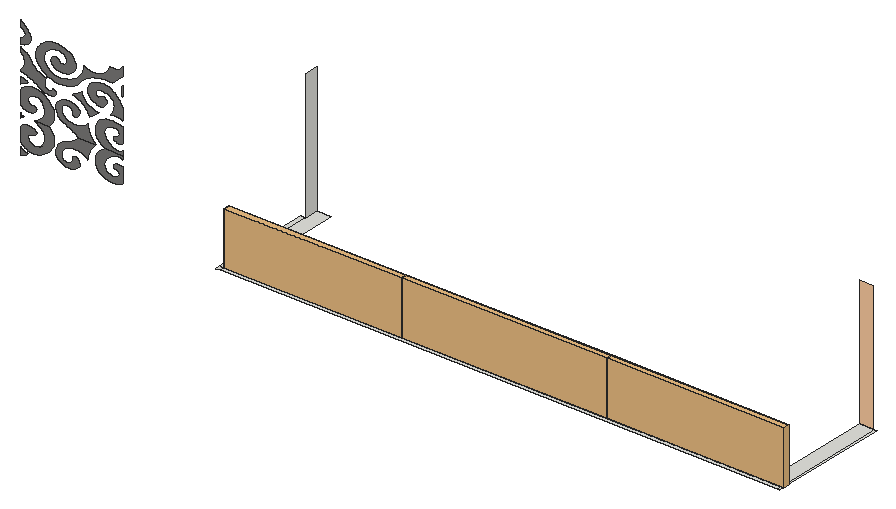
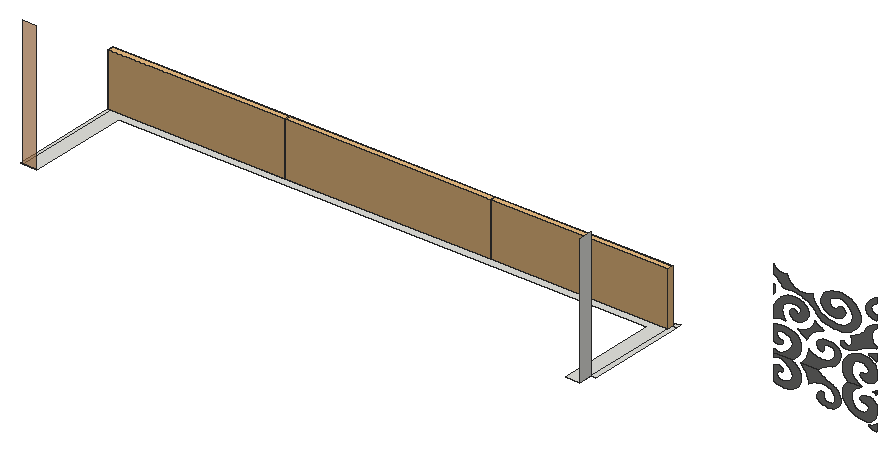
# SketchUp Ruby script. Lengths in inches.
U = 1.inch
M = Sketchup.active_model
def pt(a) = Geom::Point3d.new(a.map { |v| v * U })
def face(e, loops, mat)
  f = e.add_face(loops[0].map { |a| pt(a) })
  loops[1..].each { |l| e.add_face(l.map { |a| pt(a) }).erase! }
  f.material = f.back_material = mat if mat
  f
end
# faces: each face lists its corners as indices into pts; further lists are holes
def faces(e, pts, list, mat = nil) = list.each { |f| face(e, (f[0].is_a?(Array) ? f : [f]).map { |l| l.map { |i| pts[i] } }, mat) }
# xy, xz, yz: faces in a plane at the given z, y or x. An outline is a flat list of corners, or four numbers for a rectangle; further outlines are holes
def ring(l) = l.size == 4 ? [[l[0], l[1]], [l[2], l[1]], [l[2], l[3]], [l[0], l[3]]] : l.each_slice(2).to_a
def flat(e, list, mat, &to3) = list.each { |f| face(e, (f[0].is_a?(Array) ? f : [f]).map { |l| ring(l).map { |u, v| to3.(u, v) } }, mat) }
def xy(e, z, list, mat = nil) = flat(e, list, mat) { |x, y| [x, y, z] }
def xz(e, y, list, mat = nil) = flat(e, list, mat) { |x, z| [x, y, z] }
def yz(e, x, list, mat = nil) = flat(e, list, mat) { |y, z| [x, y, z] }
def lines(e, pts, list) = list.each { |a, b| e.add_line(pt(pts[a]), pt(pts[b])) }
# prism: a flat outline (further loops are holes) pulled along v
def prism(e, loops, v, mat = nil)
  f = face(e, loops, mat); d = Geom::Vector3d.new(v.map { |x| x * U })
  f.pushpull(f.normal.samedirection?(d) ? d.length : -d.length)
end
def box(e, o, s, mat = nil) = prism(e, [[o, [o[0] + s[0], o[1], o[2]], [o[0] + s[0], o[1] + s[1], o[2]], [o[0], o[1] + s[1], o[2]]]], [0, 0, s[2]], mat)
def at(x, y, z, deg = 0) = Geom::Transformation.translation(pt([x, y, z])) * Geom::Transformation.rotation(ORIGIN, Z_AXIS, deg.degrees)
def axes(o, x, y, z) = Geom::Transformation.new([*x, 0, *y, 0, *z, 0, *pt(o).to_a, 1])
def part(name) = M.definitions.add(name)
# library, detail: a bought-in or finely detailed component or shape, given as its bounding box
def library(name, o, s) = part(name).tap { |d| box(d.entities, o, s) }
def detail(e, o, s) = box(e.add_group.entities, o, s)
def put(e, d, t, mat = nil) = e.add_instance(d, t).tap { |i| i.material = mat if mat }
def group(e, t, mat = nil) = e.add_group.tap { |g| g.transformation = t; g.material = mat if mat }.entities
root = M.entities
M.materials.add("[0043_SaddleBrown]4").color = [124, 123, 122]
M.materials.add("[Granite Light Gray]").color = [149, 148, 144]
M.materials.add("[Wood Floor]").color = [224, 152, 88]
M.materials["[Wood Floor]"].alpha = 0.68
c1 = library("Glass Railing",[0,0,0],[139.5,4.76,42])
xy(root,293,[[548.32,556.4375,551.76,559.875],[551.76,556.4375,990.19,559.875],[990.19,556.4375,992.12,559.875],[548.32,559.875,551.76,640.11],[551.76,559.875,990.19,559.875,990.19,651.03,978.86,651.03,978.86,571.2,563.08,571.2,563.08,651.03,551.76,651.03],
  [990.19,559.875,992.12,651.03]])
xz(root,589.17,[[367.98,295.77,367.98,301,368.33,300.64,368.72,300.3,369.14,299.98,369.59,299.68,370.0625,299.4,370.5625,299.15,371.09,298.92,371.63,298.72,372.19,298.54,372.77,298.4,373.36,298.28,373.96,298.1875,373.59,297.86,373.19,297.54,372.77,297.25,372.3125,296.98,371.83,296.74,371.33,296.52,370.8,296.32,370.26,296.15,369.71,296.02,369.14,295.91,368.56,295.82],[405.94,299.46,403.95,299.6,402.04,300.03,400.29,300.72,398.77,301.66,397.55,302.81,396.67,304.1,396.18,305.5,396.03,306.54,396.01,307.57,396.12,308.61,396.34,309.63,396.7,310.64,397.17,311.62,397.76,312.57,398.46,313.47,399.27,314.33,400.18,315.14,401.19,315.88,402.28,316.56,403.43,316.875,404.56,317.24,405.66,317.65,406.72,318.1,407.74,318.59,408.73,319.13,409.67,319.7,410.57,320.3125,411.42,320.96,412.21,321.64,412.96,322.35,413.64,323.09,427.41,323.09,426.43,322.2,425.52,321.27,424.7,320.31,423.96,319.31,423.31,318.28,422.75,317.22,422.28,316.14,421.9,315.03,421.61,313.92,421.43,312.79,421.33,311.66,421.34,310.53,420.76,311.07,420.125,311.58,419.44,312.0625,418.72,312.51,417.95,312.91,417.14,313.28,416.31,313.6,415.4375,313.88,414.54,314.11,413.625,314.3,412.7,314.44,411.75,314.54,410.125,314.5625,408.51,314.41,406.96,314.07,405.49,313.56,404.16,312.89,402.99,312.07,402.01,311.14,401.24,310.1,400.71,308.99,400.43,307.84,400.41,306.66,400.64,305.5,400.9,304.93,401.29,304.41,401.81,303.9375,402.4375,303.54,403.15,303.24,403.9375,303.04,404.76,302.93,405.59,302.94,406.4,303.06,407.18,303.28,407.88,303.6,408.5,304,408.66,304.24,408.8,304.5,408.92,304.75,409.03,305.01,409.11,305.28,409.17,305.54,409.21,305.8125,409.24,306.08,409.24,306.36,409.22,306.625,409.18,306.9,409.12,307.16,409.08,307.41,409.11,307.66,409.19,307.9,409.33,308.13,409.52,308.34,409.76,308.52,410.04,308.67,410.35,308.78,410.68,308.85,411.03,308.875,411.37,308.86,411.71,308.8,412.31,308.46,412.87,308.07,413.35,307.64,413.77,307.17,414.12,306.68,414.39,306.15,414.58,305.61,414.69,305.0625,414.71,304.51,414.66,303.95,414.51,303.41,414.29,302.875,413.08,301.72,411.58,300.77,409.84,300.06,407.93,299.61],[378.81,299.94,377.24,299.97,375.69,300.16,374.2,300.52,372.81,301.04,371.54,301.7,370.43,302.5,369.49,303.41,368.76,304.41,368.25,305.48,367.98,306.59,367.98,314.54,368.4375,315.41,369.12,316.19,369.99,316.875,371.02,317.42,372.18,317.82,373.43,318.05,374.71,318.11,375.98,318,377.21,317.71,378.33,317.27,379.32,316.67,380.13,315.96,380.375,315.64,380.53,315.29,380.6,314.93,380.58,314.57,380.47,314.22,380.27,313.88,379.99,313.58,379.64,313.32,379.23,313.11,378.77,312.96,378.28,312.86,377.78,312.84,377.11,312.8,376.47,312.6875,375.86,312.49,375.3,312.23,374.82,311.89,374.42,311.51,374.125,311.08,373.93,310.62,373.86,310.14,373.9,309.66,374.05,309.1875,374.31,308.75,374.69,307.98,375.26,307.28,376.01,306.67,376.9,306.17,377.91,305.8,378.99,305.58,380.12,305.5,381.24,305.58,382.32,305.81,383.32,306.18,384.75,307.48,385.88,308.92,386.69,310.46,387.16,312.08,387.29,313.73,387.0625,315.38,386.49,316.98,385.58,318.5,384.37,319.9,382.86,321.15,381.12,322.22,379.16,323.09,390.11,323.09,391.93,321.23,393.33,319.18,394.26,317,394.7,314.75,394.64,312.47,394.09,310.22,393.05,308.07,391.55,306.0625,389.625,304.25,387.33,302.68,384.72,301.39,381.87,300.42,380.36,300.1],[440.64,301.35,437.94,301.57,435.35,302.17,432.97,303.12,430.9,304.39,429.22,305.93,427.99,307.67,427.26,309.5625,427.06,311.52,427.4,313.46,427.48,314.46,427.68,315.44,428.01,316.41,428.46,317.35,429.03,318.26,429.71,319.125,430.49,319.94,431.38,320.71,432.36,321.41,433.43,322.04,434.57,322.6,435.77,323.09,448.37,323.09,448.37,320.125,448.07,320.4,447.72,320.65,447.34,320.87,446.92,321.05,446.48,321.2,446.02,321.3,445.54,321.37,445.06,321.4,444.57,321.38,444.09,321.32,443.62,321.23,443.17,321.09,442.09,320.67,441.06,320.19,440.07,319.66,439.15,319.08,438.28,318.45,437.47,317.78,436.74,317.07,436.08,316.33,435.5,315.55,434.99,314.74,434.57,313.91,434.23,313.06,434.03,312.23,434,311.39,434.14,310.55,434.45,309.74,434.91,308.97,435.53,308.25,436.28,307.61,437.15,307.05,438.13,306.59,439.1875,306.24,440.31,306,441.46,305.875,442.53,305.92,443.55,306.14,444.46,306.54,445.21,307.09,445.75,307.75,446.04,308.49,446.08,309.26,445.86,310.01,445.39,310.7,444.7,311.28,443.84,311.73,442.85,312.01,442.6,312,442.35,312.01,442.12,312.06,441.89,312.13,441.6875,312.23,441.51,312.36,441.37,312.5,441.26,312.66,441.19,312.83,441.17,313.01,441.18,313.18,441.24,313.36,441.53,313.84,441.92,314.28,442.4,314.67,442.97,315,443.6,315.25,444.28,315.43,444.99,315.53,445.72,315.54,446.4375,315.47,447.13,315.3125,447.78,315.08,448.37,314.77,448.37,302.99,445.96,302.08,443.35,301.53],[367.98,321.36,367.98,323.09,370.37,323.09,370.06,323.07,369.75,323.03,369.46,322.96,369.17,322.86,368.91,322.73,368.68,322.58,368.47,322.41,368.3,322.22,368.16,322.02,368.06,321.81,368,321.59],
  [367.98,323.09,370.37,323.09,370.06,323.1,369.75,323.15,369.46,323.22,369.17,323.32,368.91,323.45,368.68,323.59,368.47,323.76,368.3,323.95,368.16,324.16,368.06,324.37,368,324.59,367.98,324.82],[379.16,323.09,390.11,323.09,391.93,324.95,393.33,326.99,394.26,329.17,394.7,331.43,394.64,333.71,394.09,335.95,393.05,338.11,391.55,340.11,389.625,341.93,387.33,343.5,384.72,344.78,381.87,345.76,380.36,346.08,378.81,346.23,377.24,346.21,375.69,346.02,374.2,345.66,372.81,345.14,371.54,344.47,370.43,343.68,369.49,342.77,368.76,341.77,368.25,340.7,367.98,339.58,367.98,331.63,368.4375,330.77,369.12,329.98,369.99,329.3,371.02,328.75,372.18,328.36,373.43,328.12,374.71,328.0625,375.98,328.18,377.21,328.46,378.33,328.91,379.32,329.5,380.13,330.22,380.375,330.54,380.53,330.88,380.6,331.24,380.58,331.61,380.47,331.96,380.27,332.29,379.99,332.6,379.64,332.86,379.23,333.07,378.77,333.22,378.28,333.3125,377.78,333.34,377.11,333.375,376.47,333.49,375.86,333.68,375.3,333.95,374.82,334.28,374.42,334.67,374.125,335.1,373.93,335.5625,373.86,336.04,373.9,336.52,374.05,336.99,374.31,337.43,374.69,338.2,375.26,338.9,376.01,339.51,376.9,340,377.91,340.375,378.99,340.6,380.12,340.68,381.24,340.6,382.32,340.37,383.32,340,384.75,338.7,385.88,337.26,386.69,335.71,387.16,334.1,387.29,332.44,387.0625,330.8,386.49,329.2,385.58,327.68,384.37,326.28,382.86,325.02,381.12,323.95],[413.64,323.09,427.41,323.09,426.43,323.97,425.52,324.9,424.7,325.87,423.96,326.87,423.31,327.9,422.75,328.96,422.28,330.04,421.9,331.14,421.61,332.26,421.43,333.38,421.33,334.51,421.34,335.65,420.76,335.11,420.125,334.59,419.44,334.11,418.72,333.67,417.95,333.27,417.14,332.9,416.31,332.58,415.4375,332.3,414.54,332.0625,413.625,331.875,412.7,331.73,411.75,331.64,410.125,331.61,408.51,331.77,406.96,332.11,405.49,332.62,404.16,333.29,402.99,334.1,402.01,335.04,401.24,336.08,400.71,337.18,400.43,338.34,400.41,339.51,400.64,340.67,400.9,341.24,401.29,341.77,401.81,342.24,402.4375,342.63,403.15,342.9375,403.9375,343.14,404.76,343.24,405.59,343.23,406.4,343.12,407.18,342.9,407.88,342.58,408.5,342.18,408.66,341.93,408.8,341.68,408.92,341.42,409.03,341.16,409.11,340.9,409.17,340.63,409.21,340.36,409.24,340.09,409.24,339.82,409.22,339.55,409.18,339.28,409.12,339.01,409.08,338.76,409.11,338.52,409.19,338.27,409.33,338.05,409.52,337.84,409.76,337.66,410.04,337.51,410.35,337.4,410.68,337.33,411.03,337.3,411.37,337.32,411.71,337.37,412.31,337.72,412.87,338.11,413.35,338.54,413.77,339,414.12,339.5,414.39,340.02,414.58,340.5625,414.69,341.11,414.71,341.67,414.66,342.22,414.51,342.77,414.29,343.3,413.08,344.45,411.58,345.41,409.84,346.12,407.93,346.5625,405.94,346.72,403.95,346.58,402.04,346.15,400.29,345.45,398.77,344.51,397.55,343.37,396.67,342.07,396.18,340.67,396.03,339.64,396.01,338.6,396.12,337.57,396.34,336.54,396.7,335.54,397.17,334.56,397.76,333.61,398.46,332.7,399.27,331.84,400.18,331.04,401.19,330.3,402.28,329.62,403.43,329.3,404.56,328.9375,405.66,328.53,406.72,328.08,407.74,327.58,408.73,327.05,409.67,326.47,410.57,325.86,411.42,325.22,412.21,324.54,412.96,323.83],[435.77,323.09,448.37,323.09,448.37,326.05,448.07,325.77,447.72,325.53,447.34,325.31,446.92,325.125,446.48,324.98,446.02,324.87,445.54,324.8,445.06,324.78,444.57,324.79,444.09,324.85,443.62,324.95,443.17,325.09,442.09,325.51,441.06,325.99,440.07,326.52,439.15,327.1,438.28,327.72,437.47,328.39,436.74,329.1,436.08,329.85,435.5,330.625,434.99,331.43,434.57,332.27,434.23,333.12,434.03,333.95,434,334.79,434.14,335.62,434.45,336.44,434.91,337.21,435.53,337.92,436.28,338.57,437.15,339.125,438.13,339.58,439.1875,339.9375,440.31,340.18,441.46,340.3,442.53,340.26,443.55,340.03,444.46,339.64,445.21,339.09,445.75,338.43,446.04,337.6875,446.08,336.92,445.86,336.17,445.39,335.48,444.7,334.89,443.84,334.45,442.85,334.17,442.6,334.18,442.35,334.17,442.12,334.12,441.89,334.05,441.6875,333.95,441.51,333.82,441.37,333.68,441.26,333.52,441.19,333.35,441.17,333.17,441.18,332.99,441.24,332.82,441.53,332.34,441.92,331.9,442.4,331.51,442.97,331.18,443.6,330.92,444.28,330.74,444.99,330.65,445.72,330.64,446.4375,330.71,447.13,330.86,447.78,331.1,448.37,331.41,448.37,343.1875,445.96,344.1,443.35,344.65,440.64,344.82,437.94,344.61,435.35,344.01,432.97,343.06,430.9,341.79,429.22,340.25,427.99,338.5,427.26,336.61,427.06,334.66,427.4,332.71,427.48,331.72,427.68,330.74,428.01,329.77,428.46,328.83,429.03,327.92,429.71,327.05,430.49,326.23,431.38,325.47,432.36,324.77,433.43,324.13,434.57,323.57],[422.53,341.21,423.06,341.68,423.61,342.15,424.16,342.61,424.72,343.0625,425.29,343.51,425.87,343.95,426.46,344.38,427.0625,344.81,427.67,345.23,428.29,345.64,428.92,346.04,429.5625,346.4375,427.89,346.72,426.28,347.12,424.73,347.65,423.27,348.29,421.92,349.05,420.6875,349.9,419.59,350.85,418.64,351.87,417.84,352.97,417.22,354.11,416.76,355.3,416.49,356.52,415.94,356.14,415.39,355.77,414.82,355.4,414.24,355.04,413.66,354.69,413.0625,354.35,412.46,354.02,411.85,353.6875,411.23,353.37,409.97,352.75,409.33,352.46,410.93,351.92,412.47,351.3,413.9375,350.58,415.32,349.79,416.62,348.92,417.8125,347.98,418.9,346.98,419.875,345.91,420.73,344.8,421.46,343.64,422.06,342.4375],
  [367.98,345.18,368.33,345.53,368.72,345.875,369.14,346.2,369.59,346.5,370.0625,346.77,370.5625,347.03,371.09,347.26,371.63,347.46,372.19,347.63,372.77,347.78,373.36,347.9,373.96,347.99,373.59,348.32,373.19,348.63,372.77,348.93,372.3125,349.19,371.83,349.44,371.33,349.66,370.8,349.85,370.26,350.02,369.71,350.16,369.14,350.27,368.56,350.35,367.98,350.4],[391.62,345.8,392.64,345.82,393.45,345.91,394.22,346.14,394.89,346.49,395.4375,346.93,395.83,347.45,396.06,348.03,396.09,348.625,395.95,349.21,395.62,349.76,395.13,350.24,394.5,350.625,393.77,350.9,393.66,350.3,393.34,349.75,392.83,349.27,392.17,348.9,391.4,348.67,390.57,348.59,389.74,348.67,388.97,348.9,388.3,349.27,387.79,349.75,387.47,350.3,387.36,350.9,387.32,351.375,387.29,351.85,387.29,352.33,387.3,352.8,387.32,353.28,387.37,353.75,387.43,354.22,387.51,354.7,387.61,355.17,387.72,355.63,387.85,356.1,388,356.5625,386.54,356.99,385.13,357.49,383.78,358.08,382.49,358.74,381.29,359.47,380.17,360.27,379.14,361.14,378.2,362.05,377.375,363.02,376.66,364.03,376.05,365.09,375.57,366.17,375.04,366.67,374.5,367.16,373.93,367.64,373.34,368.1,372.73,368.55,372.11,368.99,371.46,369.41,370.8,369.82,370.12,370.21,369.42,370.59,368.7,370.95,367.98,371.29,367.98,368.08,368.99,367.17,369.85,366.18,370.53,365.12,371.02,364.01,371.32,362.86,371.42,361.69,371.32,360.52,371.02,359.375,370.53,358.26,369.85,357.2,368.99,356.21,367.98,355.3,367.98,354.25,369.26,354.05,370.53,353.81,371.79,353.53,373.02,353.19,374.22,352.8125,375.39,352.39,376.54,351.92,377.64,351.4,378.71,350.85,379.74,350.26,380.72,349.63,381.65,348.96,382.38,348.45,383.16,347.98,383.98,347.55,384.84,347.16,385.74,346.82,386.67,346.53,387.625,346.28,388.6,346.08,389.6,345.9375,390.61,345.85],[448.37,347.78,448.37,356.71,448,357.36,447.62,358,447.23,358.64,446.8125,359.27,446.39,359.9,445.95,360.52,445.49,361.13,445.02,361.74,444.53,362.35,444.03,362.95,443.51,363.54,442.98,364.12,442.125,364.94,441.14,365.6875,440.05,366.34,438.85,366.9,437.58,367.36,436.24,367.71,434.85,367.94,433.4375,368.0625,432.01,368.0625,430.6,367.94,429.21,367.71,427.87,367.36,425.9375,366.59,424.24,365.57,422.86,364.33,421.82,362.92,421.19,361.39,420.98,359.81,421.19,358.23,421.82,356.7,422.86,355.29,424.24,354.05,425.9375,353.03,427.87,352.26,428.51,351.99,429.21,351.8,429.93,351.6875,430.67,351.66,431.41,351.71,432.13,351.86,432.81,352.08,433.43,352.37,433.98,352.73,434.4375,353.15,434.8,353.62,435.06,354.12,435.42,354.57,435.7,355.05,435.875,355.55,435.95,356.0625,435.93,356.58,435.8,357.09,435.58,357.59,435.26,358.05,434.85,358.48,434.37,358.86,433.8125,359.19,433.2,359.46,432.84,359.32,432.5,359.17,432.18,359,431.87,358.82,431.58,358.62,431.31,358.41,431.06,358.18,430.83,357.94,430.625,357.69,430.44,357.43,430.29,357.17,430.16,356.89,429.4,357.23,428.73,357.65,428.19,358.17,427.78,358.74,427.54,359.36,427.45,360,427.54,360.64,427.78,361.26,428.19,361.84,428.73,362.35,429.4,362.78,430.16,363.11,431.09,363.13,432.03,363.11,432.95,363.03,433.87,362.91,434.77,362.73,435.66,362.51,436.51,362.24,437.34,361.93,438.13,361.57,438.88,361.17,439.59,360.73,440.25,360.26,440.84,359.34,441.3,358.39,441.65,357.41,441.875,356.41,441.97,355.41,441.94,354.4,441.79,353.39,441.51,352.4,441.11,351.4375,440.59,350.5,439.96,349.6,439.21,348.74,439.98,348.93,440.76,349.07,441.55,349.17,442.36,349.21,443.16,349.2,443.97,349.14,444.76,349.03,445.54,348.875,446.29,348.67,447.02,348.42,447.71,348.12],[398.65,356.35,401.81,356.47,404.89,356.98,407.8125,357.86,410.49,359.07,412.84,360.6,414.79,362.39,415.33,363.14,415.92,363.86,416.56,364.5625,417.24,365.25,417.97,365.9,418.73,366.53,419.54,367.14,420.39,367.72,421.27,368.26,422.19,368.78,423.14,369.26,424.125,369.72,425.43,370.16,426.76,370.56,428.125,370.9,429.51,371.18,430.92,371.41,432.34,371.59,433.77,371.7,435.21,371.76,436.65,371.77,438.09,371.71,439.53,371.6,440.95,371.43,442.07,372.71,442.65,373.34,443.24,373.96,443.85,374.58,444.46,375.19,445.08,375.8,445.72,376.4,446.36,376.99,447.02,377.58,447.6875,378.16,448.37,378.74,448.37,385.48,448,384.78,447.5,384.13,446.88,383.54,446.15,383.01,445.33,382.5625,444.43,382.2,443.46,381.9375,442.45,381.77,441.43,381.71,440.4,381.75,439.38,381.9,438.41,382.14,437.97,380.54,437.15,379.02,435.99,377.62,434.51,376.38,432.76,375.35,430.79,374.54,428.66,373.99,426.43,373.7,424.16,373.7,421.93,373.98,419.79,374.52,417.82,375.32,417.76,373.3,417.29,371.31,416.43,369.39,415.1875,367.57,413.6,365.91,411.68,364.43,409.5,363.17,407.08,362.14,404.48,361.39,401.75,360.91,398.96,360.72,396.16,360.82,393.71,361.55,391.5,362.6,389.61,363.94,388.11,365.52,387.07,367.27,386.51,369.14,386.47,371.05,386.9375,372.94,387.9,374.72,389.32,376.33,391.15,377.71,393.3125,378.82,394.71,379.26,396.2,379.49,397.72,379.5,399.22,379.28,400.62,378.85,401.87,378.22,402.92,377.42,403.71,376.48,404.23,375.45,404.44,374.36,404.35,373.26,403.94,372.2,403.66,371.81,403.29,371.47,402.82,371.19,402.29,370.98,401.71,370.85,401.11,370.81,400.5,370.85,399.92,370.98,399.39,371.19,398.93,371.47,398.55,371.81,398.27,372.2,398.14,372.43,397.98,372.65,397.79,372.85,397.58,373.05,397.35,373.23,397.1,373.4,396.83,373.55,396.55,373.6875,396.25,373.81,395.93,373.91,395.61,373.99,395.28,374.05,394.7,373.81,394.17,373.51,393.69,373.17,393.27,372.79,392.91,372.37,392.64,371.93,392.43,371.47,392.3125,370.99,392.27,370.5,392.32,370.02,392.44,369.54,392.65,369.08,393.04,368.45,393.52,367.87,394.08,367.32,394.73,366.82,395.44,366.37,396.22,365.98,397.05,365.65,397.92,365.39,398.83,365.2,399.76,365.08,400.7,365.03,401.65,365.05,403.14,365.22,404.59,365.53,405.97,365.98,407.25,366.56,408.41,367.25,409.44,368.05,410.3,368.95,411,369.91,411.51,370.9375,411.82,372,411.9375,373.09,411.85,374.18,411.25,375.81,410.32,377.37,409.1,378.8125,407.61,380.12,405.88,381.26,403.9375,382.21,401.83,382.95,399.6,383.47,397.28,383.76,394.9375,383.8,392.6,383.61,390.34,383.18,388.14,382.09,386.16,380.8125,384.42,379.36,382.97,377.75,381.81,376.03,380.97,374.21,380.46,372.32,380.3,370.41,380.48,368.5,381,366.62,381.86,364.8,383.04,363.08,384.84,361.21,387.06,359.58,389.63,358.25,392.47,357.25,395.51,356.61],[448.37,364.66,448.37,371.94,448.14,371.35,447.96,370.75,447.8125,370.14,447.71,369.53,447.65,368.92,447.625,368.3,447.65,367.69,447.71,367.07,447.8125,366.46,447.96,365.85,448.14,365.25],
  [367.98,373.83,369.22,373.9,370.44,374.11,371.61,374.45,372.68,374.91,373.65,375.49,374.49,376.16,375.17,376.92,375.6875,377.74,376.03,378.61,376.18,379.51,376.14,380.41,375.91,381.3,375.5625,382.16,375.15,383.01,374.68,383.84,374.15,384.65,373.56,385.45,372.91,386.22,372.22,386.96,371.46,387.68,370.66,388.36,369.8125,389.02,368.92,389.64,367.98,390.23,367.98,385.49,369.06,385.16,370.02,384.67,370.82,384.05,371.42,383.32,371.79,382.52,371.92,381.67,371.79,380.83,371.42,380.02,370.82,379.29,370.02,378.67,369.06,378.18,367.98,377.85]],"[0043_SaddleBrown]4")
xz(root,651.03,[[978.86,293,990.19,394.4375]],"[Wood Floor]")
yz(root,551.76,[[640.11,293,651.03,394.4375]])
p = [[383.32,589.17,306.18],[384.21,589.17,306.68],[384.96,589.17,307.29],[383.32,589.17,340],[384.21,589.17,339.5],[384.96,589.17,338.89]]
lines(root,p,[[0,1],[1,2],[3,4],[4,5]])
put(root,c1,at(551.76,559.875,293))
put(root,c1,axes([691.26,559.875,293],[1.15726,0,0],[0,1,0],[0,0,1]),"[Granite Light Gray]")
put(root,c1,at(852.7,559.875,293))
